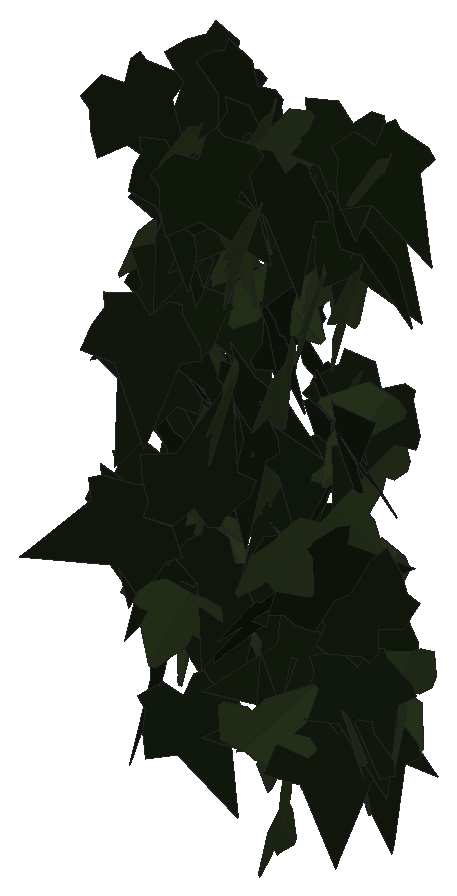
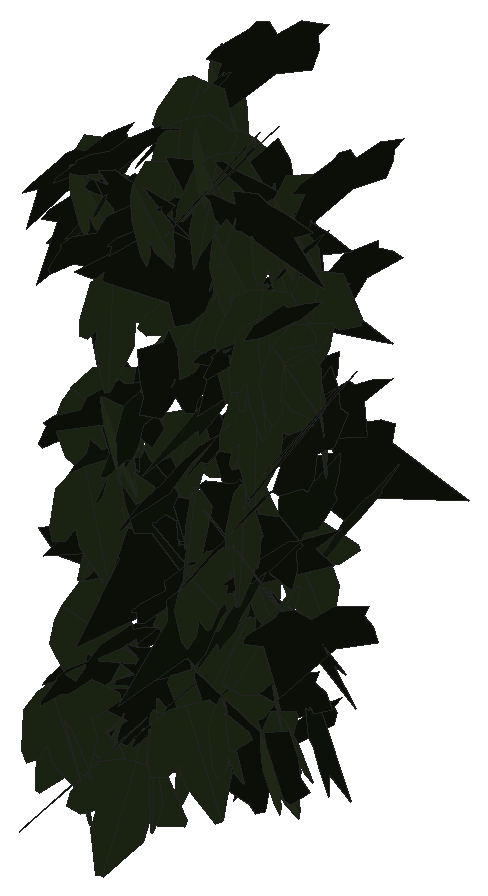
# SketchUp Ruby script. Lengths in inches.
U = 1.inch
M = Sketchup.active_model
def pt(a) = Geom::Point3d.new(a.map { |v| v * U })
def face(e, loops, mat)
  f = e.add_face(loops[0].map { |a| pt(a) })
  loops[1..].each { |l| e.add_face(l.map { |a| pt(a) }).erase! }
  f.material = f.back_material = mat if mat
  f
end
# faces: each face lists its corners as indices into pts; further lists are holes
def faces(e, pts, list, mat = nil) = list.each { |f| face(e, (f[0].is_a?(Array) ? f : [f]).map { |l| l.map { |i| pts[i] } }, mat) }
# xy, xz, yz: faces in a plane at the given z, y or x. An outline is a flat list of corners, or four numbers for a rectangle; further outlines are holes
def ring(l) = l.size == 4 ? [[l[0], l[1]], [l[2], l[1]], [l[2], l[3]], [l[0], l[3]]] : l.each_slice(2).to_a
def flat(e, list, mat, &to3) = list.each { |f| face(e, (f[0].is_a?(Array) ? f : [f]).map { |l| ring(l).map { |u, v| to3.(u, v) } }, mat) }
def xy(e, z, list, mat = nil) = flat(e, list, mat) { |x, y| [x, y, z] }
def xz(e, y, list, mat = nil) = flat(e, list, mat) { |x, z| [x, y, z] }
def yz(e, x, list, mat = nil) = flat(e, list, mat) { |y, z| [x, y, z] }
def lines(e, pts, list) = list.each { |a, b| e.add_line(pt(pts[a]), pt(pts[b])) }
# prism: a flat outline (further loops are holes) pulled along v
def prism(e, loops, v, mat = nil)
  f = face(e, loops, mat); d = Geom::Vector3d.new(v.map { |x| x * U })
  f.pushpull(f.normal.samedirection?(d) ? d.length : -d.length)
end
def box(e, o, s, mat = nil) = prism(e, [[o, [o[0] + s[0], o[1], o[2]], [o[0] + s[0], o[1] + s[1], o[2]], [o[0], o[1] + s[1], o[2]]]], [0, 0, s[2]], mat)
def at(x, y, z, deg = 0) = Geom::Transformation.translation(pt([x, y, z])) * Geom::Transformation.rotation(ORIGIN, Z_AXIS, deg.degrees)
def axes(o, x, y, z) = Geom::Transformation.new([*x, 0, *y, 0, *z, 0, *pt(o).to_a, 1])
def part(name) = M.definitions.add(name)
# library, detail: a bought-in or finely detailed component or shape, given as its bounding box
def library(name, o, s) = part(name).tap { |d| box(d.entities, o, s) }
def detail(e, o, s) = box(e.add_group.entities, o, s)
def put(e, d, t, mat = nil) = e.add_instance(d, t).tap { |i| i.material = mat if mat }
def group(e, t, mat = nil) = e.add_group.tap { |g| g.transformation = t; g.material = mat if mat }.entities
root = M.entities
M.materials.add("efeu1").color = [18, 25, 13]
M.materials.add("efeu2").color = [43, 57, 29]
c1 = part("ivyleaf_9")
p = [[1.54,2.16,1.25],[1.36,2.04,1.19],[-0.21,0.99,0.68],[-0.71,1.11,0.82],[-0.85,0.86,0.67],[-0.8,0.17,0.21],
  [-0.9,-0.01,0.1],[-0.67,-0.16,-0.02],[-0.08,-0.08,-0.05],[-0.03,-0.6,-0.4],[0.65,-0.88,-0.66],[0.83,-0.6,-0.49],
  [1.29,-0.42,-0.43],[1.8125,-0.07,-0.26],[1.21,0.44,0.15]]
faces(c1.entities,p,[[0,1,2,3,4,5,6,7,8,9,10,11,12,13,14]],"efeu1")
c2 = part("ivyleaf_10")
p = [[0,0.5,-0.03],[-0.0625,2.02,-0.43],[-0.19,2.01,-0.46],[-0.54,1.05,-0.29],[-0.52,0.625,-0.18],[-0.83,0.76,-0.28],
  [-1.16,0.64,-0.33],[-1.15,0.33,-0.24],[-0.77,-0.39,0.02],[-0.3,-0.51,0.16],[0.04,-0.48,0.23],[-0.02,2.01,-0.4375],
  [-0.06,2.01,-0.43],[0.04,-0.49,0.23],[0.67,-0.49,0.14],[1.38,0.36,-0.2],[1.375,0.51,-0.24],[0.81,0.65,-0.19],
  [0.62,0.59,-0.15],[0.6,1.09,-0.28],[0.5,1.23,-0.31]]
faces(c2.entities,p,[[0,1,2,3,4,5,6,7,8,9,10],[11,12,0,13,14,15,16,17,18,19,20]],"efeu2")
put(root,c1,axes([30.6,221.93,236.72],[-0.10073,-0.4149,-0.26021],[0.09758,0.24333,-0.42575],[0.47993,-0.13655,0.03195]))
put(root,c1,axes([30.62,221.18,241.97],[0.14716,-0.365,-0.30841],[-0.02814,0.31553,-0.38685],[0.47702,0.13121,0.07232]))
put(root,c2,axes([30.83,222.09,239.86],[-0.02241,-0.41383,0.27972],[0.09339,-0.27854,-0.40459],[0.49069,0.03412,0.08978]))
put(root,c1,axes([30.6875,221.98,239.02],[0.01908,-0.45016,0.21678],[0.03566,-0.21516,-0.44993],[0.49836,0.03263,0.02389]))
put(root,c2,axes([30.97,222.32,240.13],[-0.0568,-0.49434,-0.04902],[0.00993,0.0482,-0.49757],[0.49666,-0.0575,0.00434]))
put(root,c1,axes([31.13,222.46,241.8],[-0.48411,-0.12089,-0.03197],[0.02934,0.01445,-0.49893],[0.12156,-0.48495,-0.00689]))
put(root,c2,axes([31,221.3,240.26],[-0.0587,-0.45384,-0.20146],[0.05317,0.19595,-0.45692],[0.49369,-0.07507,0.02526]))
put(root,c1,axes([30.78,222.07,238.8],[0.20523,-0.45558,-0.01825],[-0.00647,0.0171,-0.49967],[0.4559,0.20532,0.00112]))
put(root,c2,axes([31.05,222.21,240.41],[-0.18126,-0.4417,-0.14848],[0.0513,0.13944,-0.47741],[0.46316,-0.1883,-0.00524]))
put(root,c2,axes([31,222.08,235.08],[0.20623,-0.41089,0.19657],[0.09187,-0.17383,-0.45972],[0.44613,0.22574,0.00379]))
put(root,c2,axes([31.24,221.02,238.99],[0.19094,-0.30626,-0.34604],[-0.165,0.30455,-0.36059],[0.43164,0.2519,0.01523]))
put(root,c1,axes([31.02,222.47,240.25],[-0.12976,-0.47039,0.10906],[-0.01823,-0.10807,-0.48784],[0.48252,-0.13058,0.0109]))
put(root,c1,axes([31.13,222.09,237.28],[-0.2425,-0.39378,0.19009],[-0.03362,-0.19993,-0.45705],[0.43596,-0.23445,0.07049]))
put(root,c1,axes([31.25,221.41,236.32],[-0.45981,0.01586,-0.19577],[0.19487,-0.02562,-0.45975],[-0.02461,-0.49909,0.01738]))
put(root,c2,axes([31.07,221.77,235.25],[0.38124,-0.24826,0.20743],[0.16869,-0.12101,-0.45486],[0.27605,0.4168,-0.00851]))
put(root,c1,axes([31.18,221.13,238.7],[-0.17694,-0.45337,0.11467],[-0.03557,-0.1092,-0.48663],[0.46629,-0.18037,0.00639]))
put(root,c2,axes([31.27,221.99,239.1],[-0.12362,-0.47732,-0.08295],[0.02326,0.07966,-0.49306],[0.48392,-0.12577,0.00251]))
put(root,c2,axes([31.27,222.14,235.99],[-0.04584,0.39712,0.30032],[0.03716,-0.29802,0.39975],[0.49651,0.05897,-0.00219]))
put(root,c2,axes([31.22,221.54,241.27],[0.16273,-0.41785,0.22117],[0.07559,-0.2079,-0.4484],[0.4667,0.17937,-0.00449]))
put(root,c1,axes([30.88,221.52,238.53],[0.1822,-0.26809,0.38069],[0.24451,-0.29281,-0.32323],[0.39625,0.30396,0.02441]))
put(root,c2,axes([31.28,222.15,237.95],[0.05248,-0.4613,-0.18559],[0.01679,0.18816,-0.46294],[0.49695,0.04236,0.03524]))
put(root,c2,axes([31.29,221.73,241.16],[0.06072,-0.49395,0.0482],[0.00734,-0.04766,-0.49767],[0.49624,0.06115,0.00147]))
put(root,c1,axes([31.25,221.09,235],[-0.31409,0.15046,-0.35876],[0.3333,-0.13374,-0.34788],[-0.20064,-0.45769,-0.01629]))
put(root,c2,axes([31.34,222.07,240.22],[0.05151,-0.49364,0.06054],[0.00006,-0.06086,-0.49628],[0.49734,0.05114,-0.00622]))
put(root,c2,axes([31.34,222.4,241.15],[0.10703,-0.45375,0.1807],[0.0262,-0.17939,-0.46598],[0.48771,0.10921,-0.01462]))
put(root,c1,axes([31.09,222.08,234.64],[-0.15176,0.09147,0.46755],[0.38127,-0.2709,0.17676],[0.28566,0.41018,0.01247]))
put(root,c1,axes([31.07,221.47,237.47],[0.08391,-0.34447,0.35256],[0.17395,-0.31393,-0.34812],[0.4612,0.18107,0.06716]))
put(root,c1,axes([31.24,221.79,240.53],[0.02466,-0.47497,0.15425],[0.02451,-0.1531,-0.47535],[0.49879,0.03101,0.01573]))
put(root,c1,axes([31.24,220.5,237],[0.0444,-0.43518,0.24218],[0.06634,-0.23581,-0.43588],[0.49359,0.07083,0.0368]))
put(root,c1,axes([31.66,222.09,237.48],[-0.47152,0.14469,-0.08209],[0.07893,-0.02262,-0.49321],[-0.14644,-0.47807,-0.00151]))
put(root,c2,axes([31.43,220.96,239.26],[0.31245,-0.36967,0.12538],[0.09468,-0.08403,-0.48371],[0.3787,0.32601,0.01749]))
put(root,c2,axes([31.52,222.12,235.32],[0.02224,-0.47539,0.15334],[0.04642,-0.15086,-0.47443],[0.49734,0.03534,0.03742]))
put(root,c1,axes([31.29,222.5,237.74],[0.11175,-0.4804,0.08205],[0.02706,-0.07794,-0.49315],[0.4866,0.11465,0.00858]))
put(root,c1,axes([31.42,222.45,236.48],[-0.1338,-0.19447,0.44077],[0.04571,-0.46052,-0.1893],[0.47959,-0.01036,0.14101]))
put(root,c1,axes([31.31,221.97,237.77],[-0.16001,-0.12134,-0.4579],[0.38729,0.24479,-0.20021],[0.27276,-0.41876,0.01565]))
put(root,c1,axes([31.81,221,239.84],[-0.42942,-0.18532,0.1768],[-0.16257,-0.06949,-0.4677],[0.19792,-0.45916,-0.00057]))
put(root,c2,axes([31.54,222.15,241.24],[-0.24852,0.42287,-0.09707],[0.03985,-0.08915,-0.49037],[-0.43203,-0.25147,0.01061]))
put(root,c1,axes([31.41,221.12,241.22],[0.07451,-0.49259,0.04248],[0.00752,-0.04183,-0.49819],[0.49436,0.07488,0.00117]))
put(root,c2,axes([31.5625,222.61,237.11],[-0.06171,-0.37361,0.32651],[0.12297,-0.33028,-0.35468],[0.4807,0.03653,0.13265]))
put(root,c1,axes([31.65,221.29,240.9],[-0.42074,-0.24135,-0.12135],[0.1032,0.06398,-0.48503],[0.24965,-0.43319,-0.00402]))
put(root,c1,axes([31.9,219.83,237.37],[-0.05885,-0.0838,-0.4894],[-0.21297,-0.44093,0.10111],[-0.44853,0.22036,0.0162]))
put(root,c1,axes([31.49,221.63,235.42],[-0.1169,-0.42152,-0.24219],[0.05354,0.23642,-0.43731],[0.48319,-0.12817,-0.01014]))
put(root,c1,axes([31.4375,222.2,238.97],[0.14585,-0.47776,0.02173],[0.00029,-0.02263,-0.49949],[0.47825,0.14572,-0.00633]))
put(root,c2,axes([31.66,221.63,236.97],[0.07967,-0.47083,0.14822],[0.04702,-0.14222,-0.47703],[0.49137,0.08995,0.02161]))
put(root,c2,axes([31.7,221.77,240.05],[-0.17039,-0.46464,-0.07125],[0.07489,0.04799,-0.49202],[0.46407,-0.17835,0.05324]))
put(root,c2,axes([31.93,222.3125,235.11],[-0.42031,-0.14748,0.22714],[-0.21398,-0.0762,-0.44543],[0.166,-0.47164,0.00094]))
put(root,c1,axes([31.59,222.29,241.82],[-0.09222,-0.39282,0.29528],[0.03699,-0.30513,-0.39437],[0.49003,-0.05089,0.08534]))
put(root,c1,axes([31.51,221.6,239.64],[0.03745,-0.39633,-0.30252],[0.09484,0.30349,-0.38587],[0.48949,-0.02848,0.0979]))
put(root,c2,axes([31.71,221.41,238.67],[-0.35265,0.29276,-0.19982],[0.1509,-0.13105,-0.45832],[-0.32073,-0.38356,0.00407]))
put(root,c1,axes([31.76,220.15,239.78],[-0.0923,-0.48572,-0.07454],[0.01165,0.07366,-0.49441],[0.49127,-0.093,-0.00228]))
put(root,c2,axes([31.99,221.85,235.36],[0.17184,0.45046,0.1325],[-0.07086,-0.1146,0.4815],[0.46416,-0.18426,0.02445]))
put(root,c1,axes([31.73,221.58,238.64],[0.08573,-0.47523,0.12963],[0.03806,-0.12479,-0.48268],[0.49112,0.09263,0.01477]))
put(root,c1,axes([31.77,220.81,234.54],[0.1196,-0.43871,-0.20791],[0.01776,0.21794,-0.44965],[0.48516,0.10017,0.06771]))
put(root,c1,axes([31.86,222.13,236.56],[0.46215,-0.11619,-0.1514],[-0.12058,0.12969,-0.46759],[0.14793,0.4687,0.09186]))
put(root,c2,axes([32.28,220.13,236.26],[-0.38681,-0.23172,0.21608],[-0.17997,-0.11995,-0.4508],[0.26075,-0.42652,0.00939]))
put(root,c2,axes([32.2,221.71,241.78],[0.17656,-0.46621,0.03837],[0.01389,-0.03577,-0.49853],[0.46758,0.17711,0.00032]))
put(root,c2,axes([32.13,221.62,241.43],[-0.09207,-0.48249,-0.09341],[0.14121,0.06505,-0.47521],[0.47072,-0.11389,0.12429]))
put(root,c2,axes([32.24,221.8125,237.41],[0.13054,-0.39718,-0.27424],[-0.01201,0.28133,-0.41317],[0.48251,0.11446,0.06391]))
put(root,c1,axes([31.98,221.92,241.51],[0.08043,-0.47504,0.13367],[0.03958,-0.12879,-0.4815],[0.4919,0.08804,0.01689]))
put(root,c1,axes([32.05,221.08,240.78],[-0.09603,-0.06337,0.48658],[0.41159,0.25954,0.11503],[-0.26716,0.42264,0.00232]))
put(root,c1,axes([32.4,221.37,241.23],[-0.48563,-0.11374,0.03507],[-0.03302,-0.0128,-0.49874],[0.11435,-0.48672,0.00492]))
put(root,c2,axes([32.28,221.08,240.83],[-0.37802,0.3163,-0.08396],[0.05341,-0.06693,-0.49261],[-0.32287,-0.38141,0.01681]))
put(root,c2,axes([32.35,221.22,240.75],[0.21701,-0.4502,0.01518],[0.00384,-0.015,-0.49976],[0.45044,0.21702,-0.00306]))
put(root,c1,axes([32.17,221.31,238.78],[0.38668,-0.24566,-0.20034],[-0.09879,0.20687,-0.44435],[0.3012,0.38322,0.11144]))
put(root,c2,axes([32.25,221.77,239.76],[-0.27135,-0.32705,-0.26345],[0.25283,0.12322,-0.41339],[0.33533,-0.35757,0.0985]))
put(root,c1,axes([32.37,221.99,238.94],[0.09023,0.26428,0.41475],[-0.23834,-0.34535,0.2719],[0.43018,-0.24677,0.06366]))
put(root,c2,axes([32.45,220.73,241.15],[-0.48519,0.11804,-0.02572],[0.0247,-0.00726,-0.49934],[-0.11825,-0.48581,0.00121]))
put(root,c1,axes([32.29,221.24,238.16],[-0.29233,-0.07788,-0.3981],[0.39622,0.05033,-0.30079],[0.08692,-0.49133,0.03229]))
put(root,c1,axes([32.33,220.98,236.4],[-0.06345,-0.44653,0.21583],[0.00043,-0.21764,-0.45015],[0.49596,-0.05694,0.028]))
put(root,c1,axes([32.46,222.01,236.5],[-0.20172,-0.39373,0.23298],[-0.06556,-0.22712,-0.44059],[0.45278,-0.2083,0.04]))
put(root,c1,axes([32.09,221.79,240.51],[0.39061,-0.04118,0.30939],[0.31206,0.06148,-0.3858],[-0.00627,0.49449,0.07373]))
put(root,c1,axes([32.41,222.12,235.07],[-0.12111,-0.40946,0.26013],[-0.00612,-0.26681,-0.42282],[0.48507,-0.1056,0.05962]))
put(root,c2,axes([32.47,222.4,241.38],[0.14916,-0.4253,0.2165],[0.09029,-0.19758,-0.45035],[0.46861,0.17344,0.01786]))
put(root,c1,axes([32.54,220.01,237.75],[-0.25797,-0.1813,0.38805],[0.33339,0.19939,0.31479],[-0.26889,0.42116,0.01802]))
put(root,c2,axes([32.72,221.85,234.56],[0.10335,-0.40044,-0.28101],[-0.05523,0.27583,-0.41336],[0.48607,0.11648,0.01278]))
put(root,c2,axes([32.64,221.58,241.64],[-0.06153,-0.49207,-0.06388],[0.10382,0.05018,-0.48652],[0.48522,-0.07314,0.096]))
put(root,c2,axes([32.72,221.24,241.97],[-0.10893,-0.40161,-0.2772],[0.0944,0.26132,-0.41569],[0.47877,-0.1429,0.0189]))
put(root,c1,axes([32.625,220.6,235.78],[-0.0676,0.46788,-0.16284],[-0.02236,0.1613,0.47274],[0.4949,0.07119,-0.00089]))
put(root,c1,axes([32.74,222.04,240.81],[-0.20135,-0.42896,0.15954],[-0.04575,-0.15455,-0.47331],[0.45537,-0.2052,0.02299]))
put(root,c1,axes([33.15,221.63,235.05],[-0.3938,-0.02851,0.30677],[-0.30616,-0.01938,-0.39483],[0.0344,-0.49881,-0.00219]))
put(root,c1,axes([32.61,221.91,237.6875],[0.04486,-0.48566,0.11009],[0.02087,-0.1086,-0.48762],[0.49755,0.04835,0.01053]))
put(root,c1,axes([33.09,222.14,241.2],[-0.49491,-0.01408,0.06973],[-0.06935,-0.01377,-0.49498],[0.01586,-0.49961,0.01167]))
put(root,c2,axes([32.85,222.21,234.07],[-0.40353,-0.27262,-0.1133],[0.08815,0.07188,-0.48689],[0.28176,-0.41293,-0.00995]))
put(root,c1,axes([32.67,219.97,242.22],[0.06864,-0.33002,-0.36929],[-0.0002,0.3728,-0.33319],[0.49527,0.04588,0.05105]))
put(root,c1,axes([32.57,221.51,239.25],[0.24311,-0.14071,-0.41364],[0.38308,-0.159,0.27923],[-0.21012,-0.45268,0.0305]))
put(root,c1,axes([32.74,221.57,236.6875],[-0.0086,-0.07497,-0.49427],[-0.03115,0.49347,-0.07431],[0.49895,0.02951,-0.01316]))
put(root,c2,axes([32.9,220.17,239.28],[0.2382,-0.43951,0.00945],[0.00418,-0.00848,-0.49991],[0.43959,0.23824,-0.00036]))
put(root,c2,axes([32.98,221.125,234.61],[-0.02602,-0.49699,0.0482],[0.00591,-0.04857,-0.4976],[0.49929,-0.02532,0.0084]))
put(root,c2,axes([32.99,222.27,239.99],[-0.07767,-0.47961,-0.11806],[0.02702,0.1152,-0.4858],[0.49319,-0.08185,0.00802]))
put(root,c1,axes([32.64,222.25,238.55],[0.21929,-0.37355,0.24975],[0.14018,-0.20717,-0.43293],[0.42692,0.25989,0.01386]))
put(root,c1,axes([33.3125,221.54,234.41],[-0.30334,-0.09114,0.38688],[-0.37273,-0.10381,-0.3167],[0.13805,-0.48054,-0.00496]))
put(root,c1,axes([33.22,221.51,237.36],[-0.32452,0.36401,-0.1104],[0.07504,-0.081,-0.48766],[-0.37291,-0.33307,-0.00205]))
put(root,c1,axes([33.01,222.51,240.85],[-0.14761,-0.47726,0.02075],[-0.00953,-0.01877,-0.49956],[0.47762,-0.14788,-0.00355]))
put(root,c2,axes([33.09,222.18,238.44],[0.23885,-0.42573,0.10819],[0.04946,-0.09631,-0.48814],[0.43647,0.24389,-0.0039]))
put(root,c1,axes([32.99,222.31,241.77],[-0.08228,-0.4929,-0.01672],[0.09527,0.00074,-0.49084],[0.48389,-0.08396,0.0938]))
put(root,c2,axes([33.26,222.34,237.56],[-0.19691,-0.45438,0.06904],[-0.01419,-0.06906,-0.495],[0.45937,-0.1969,0.0143]))
put(root,c1,axes([33,221.09,241.66],[0.09717,-0.48795,0.04967],[0.01242,-0.04817,-0.49752],[0.49031,0.09792,0.00276]))
put(root,c2,axes([33.29,222.49,236.07],[-0.08802,-0.32014,0.37385],[-0.01325,-0.3781,-0.3269],[0.49201,-0.06745,0.05808]))
put(root,c2,axes([33.08,220.49,234.625],[-0.28376,-0.29227,0.28993],[0.20584,0.20423,0.40733],[-0.35653,0.35053,0.00442]))
put(root,c2,axes([33.25,220.125,241.55],[0.19241,-0.44125,0.13521],[0.04897,-0.12614,-0.48134],[0.45889,0.19847,-0.00533]))
put(root,c1,axes([33.0625,222.13,234.46],[0.34637,-0.25028,-0.25959],[-0.08133,0.29646,-0.39433],[0.3513,0.3154,0.16466]))
put(root,c2,axes([33.17,221.42,234.64],[0.41555,0.24796,0.12581],[0.10551,0.06871,-0.48389],[-0.25726,0.42871,0.00478]))
put(root,c1,axes([33.21,222.41,235.54],[-0.0495,-0.49602,0.03897],[0.00048,-0.03921,-0.49846],[0.49754,-0.04931,0.00436]))
put(root,c2,axes([33.43,220.43,233.81],[0.1003,-0.36524,-0.3264],[-0.02946,0.32807,-0.37616],[0.48895,0.09469,0.04429]))
put(root,c2,axes([33.41,221.12,240.33],[0.26444,-0.42432,-0.00486],[-0.00801,0.00073,-0.49994],[0.42428,0.26448,-0.00641]))
put(root,c2,axes([33.41,222.26,241.32],[0.16054,-0.44125,0.17182],[0.05508,-0.1628,-0.46954],[0.47031,0.16969,-0.00367]))
put(root,c1,axes([33.39,222.29,238.47],[-0.20192,-0.45141,0.07386],[-0.02184,-0.07112,-0.49443],[0.45689,-0.2029,0.009]))
put(root,c2,axes([33.4,221.625,237.18],[-0.0594,-0.40125,-0.29236],[0.13084,0.27138,-0.39904],[0.47891,-0.12391,0.07276]))
put(root,c2,axes([33.54,222.04,238.39],[-0.15529,-0.3336,0.33852],[-0.02627,-0.34956,-0.35653],[0.47455,-0.12852,0.09104]))
put(root,c2,axes([33.47,220.41,237.29],[-0.17522,-0.40109,-0.2417],[0.0886,0.22501,-0.43763],[0.45983,-0.1962,-0.00778]))
put(root,c1,axes([33.2,221.66,238.03],[-0.03623,0.01797,0.49836],[0.2801,-0.41267,0.03524],[0.41259,0.28174,0.01983]))
put(root,c2,axes([33.61,222.22,234.44],[0.14664,0.35742,-0.3174],[-0.22934,-0.23869,-0.37474],[-0.41941,0.25549,0.09394]))
put(root,c2,axes([33.6,222.47,234.88],[-0.16042,-0.45619,0.12711],[-0.00874,-0.13133,-0.48237],[0.47348,-0.15699,0.03416]))
put(root,c1,axes([33.24,222.04,237.75],[0.39321,-0.15158,-0.26908],[0.25393,-0.08928,0.42136],[-0.17579,-0.46803,0.00677]))
put(root,c1,axes([33.36,222.32,241.61],[0.13258,-0.43305,-0.21186],[0.00342,0.22057,-0.44871],[0.48209,0.11753,0.06145]))
put(root,c1,axes([33.39,221.89,240.93],[0.09048,-0.35556,-0.33969],[-0.0117,0.34374,-0.36292],[0.49161,0.07362,0.05388]))
put(root,c1,axes([33.46,220.86,236.76],[0.03954,0.16454,-0.47049],[-0.06061,0.47005,0.15929],[0.49474,0.04444,0.05711]))
put(root,c2,axes([33.67,222.23,234.41],[0.36825,-0.32598,-0.09016],[-0.06671,0.06067,-0.4918],[0.33157,0.37424,0.00119]))
put(root,c1,axes([34,221.45,236.04],[-0.05484,0.08784,0.48916],[-0.46643,0.16079,-0.08117],[-0.17156,-0.46522,0.06431]))
put(root,c1,axes([33.36,221.97,240.96],[0.27823,-0.41544,0.00003],[0.01981,0.01323,-0.49943],[0.41497,0.27791,0.02382]))
put(root,c2,axes([33.7,220.15,239.77],[0.11712,-0.45334,-0.1754],[-0.006,0.17906,-0.4668],[0.48605,0.11145,0.0365]))
put(root,c2,axes([33.75,221.36,240.38],[0.20959,-0.43647,0.12478],[0.07046,-0.10449,-0.48386],[0.44845,0.2204,0.01771]))
put(root,c2,axes([33.69,221.32,234.64],[-0.3327,0.33284,-0.16889],[0.12216,-0.11668,-0.4706],[-0.35268,-0.3544,-0.00368]))
put(root,c1,axes([33.65,221.6,235.21],[0.02229,-0.47467,-0.15555],[0.03068,0.15671,-0.47382],[0.49856,0.01158,0.03611]))
put(root,c1,axes([33.66,221.82,234.42],[0.07758,-0.48851,-0.07311],[-0.0126,0.07202,-0.49463],[0.49378,0.07858,-0.00113]))
put(root,c1,axes([33.75,221.08,234.6],[-0.22472,-0.39639,-0.20586],[0.08682,0.18729,-0.4554],[0.43814,-0.24042,-0.01535]))
